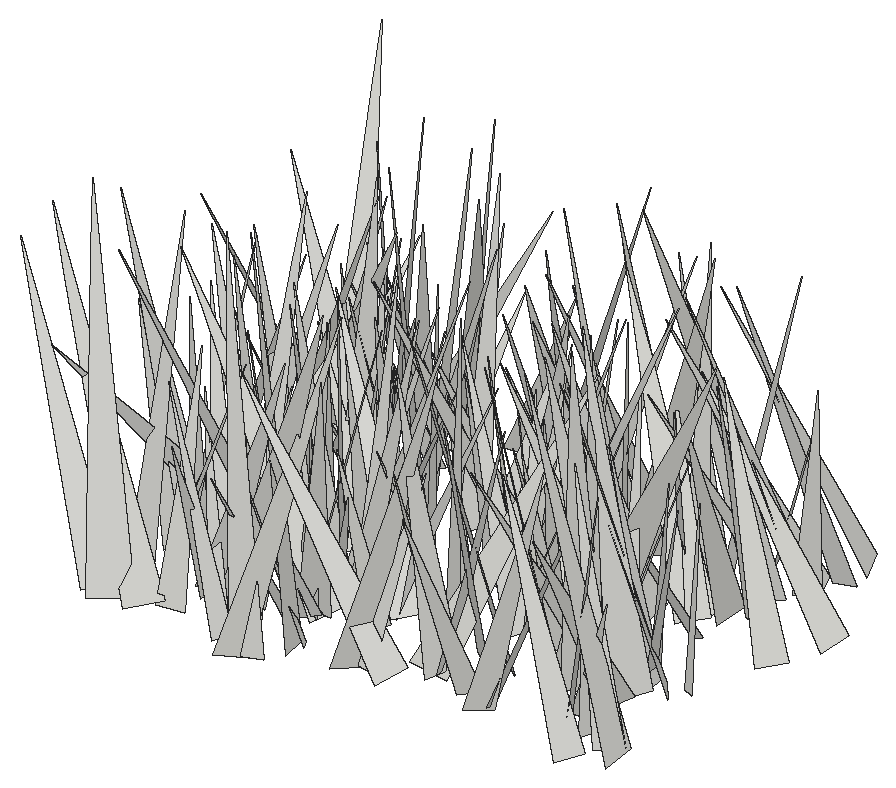
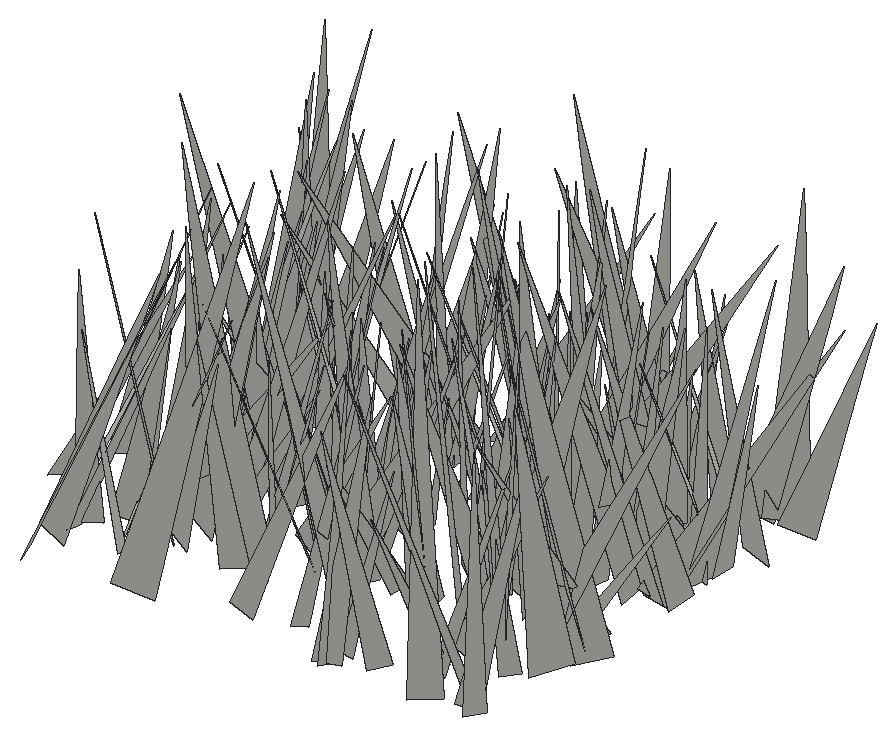
# SketchUp Ruby script. Lengths in inches.
U = 1.inch
M = Sketchup.active_model
def pt(a) = Geom::Point3d.new(a.map { |v| v * U })
def face(e, loops, mat)
  f = e.add_face(loops[0].map { |a| pt(a) })
  loops[1..].each { |l| e.add_face(l.map { |a| pt(a) }).erase! }
  f.material = f.back_material = mat if mat
  f
end
# faces: each face lists its corners as indices into pts; further lists are holes
def faces(e, pts, list, mat = nil) = list.each { |f| face(e, (f[0].is_a?(Array) ? f : [f]).map { |l| l.map { |i| pts[i] } }, mat) }
# xy, xz, yz: faces in a plane at the given z, y or x. An outline is a flat list of corners, or four numbers for a rectangle; further outlines are holes
def ring(l) = l.size == 4 ? [[l[0], l[1]], [l[2], l[1]], [l[2], l[3]], [l[0], l[3]]] : l.each_slice(2).to_a
def flat(e, list, mat, &to3) = list.each { |f| face(e, (f[0].is_a?(Array) ? f : [f]).map { |l| ring(l).map { |u, v| to3.(u, v) } }, mat) }
def xy(e, z, list, mat = nil) = flat(e, list, mat) { |x, y| [x, y, z] }
def xz(e, y, list, mat = nil) = flat(e, list, mat) { |x, z| [x, y, z] }
def yz(e, x, list, mat = nil) = flat(e, list, mat) { |y, z| [x, y, z] }
def lines(e, pts, list) = list.each { |a, b| e.add_line(pt(pts[a]), pt(pts[b])) }
# prism: a flat outline (further loops are holes) pulled along v
def prism(e, loops, v, mat = nil)
  f = face(e, loops, mat); d = Geom::Vector3d.new(v.map { |x| x * U })
  f.pushpull(f.normal.samedirection?(d) ? d.length : -d.length)
end
def box(e, o, s, mat = nil) = prism(e, [[o, [o[0] + s[0], o[1], o[2]], [o[0] + s[0], o[1] + s[1], o[2]], [o[0], o[1] + s[1], o[2]]]], [0, 0, s[2]], mat)
def at(x, y, z, deg = 0) = Geom::Transformation.translation(pt([x, y, z])) * Geom::Transformation.rotation(ORIGIN, Z_AXIS, deg.degrees)
def axes(o, x, y, z) = Geom::Transformation.new([*x, 0, *y, 0, *z, 0, *pt(o).to_a, 1])
def part(name) = M.definitions.add(name)
# library, detail: a bought-in or finely detailed component or shape, given as its bounding box
def library(name, o, s) = part(name).tap { |d| box(d.entities, o, s) }
def detail(e, o, s) = box(e.add_group.entities, o, s)
def put(e, d, t, mat = nil) = e.add_instance(d, t).tap { |i| i.material = mat if mat }
def group(e, t, mat = nil) = e.add_group.tap { |g| g.transformation = t; g.material = mat if mat }.entities
root = M.entities
c1 = part("fur_instance\#9")
p = [[0.8125,0,1.79],[0.67,-0.02,1.48],[0,-0.11,0],[0,0.11,0]]
faces(c1.entities,p,[[0,1,2,3]])
put(root,c1,axes([64.84,431.83,-27.1],[-3.24359,5.98487,0.42852],[5.75195,2.96279,2.1587],[-1.708,-1.38792,6.45597]))
put(root,c1,axes([65.26,437.11,-27.1],[-7.08698,0.49693,1.41438],[0.58095,7.2106,0.37757],[1.38199,-0.48283,7.09434]))
put(root,c1,axes([66.96,431.76,-27.1],[-3.17251,7.14398,0.8627],[6.87917,2.73438,2.65436],[-2.11131,-1.82544,7.35225]))
put(root,c1,axes([65.07,435.94,-27.1],[-4.79431,0.50788,0.77321],[0.45097,4.84644,-0.38709],[0.80772,0.30866,4.80557]))
put(root,c1,axes([65.37,445.7,-27.1],[-6.50457,4.89284,0.5628],[4.72218,6.46057,-1.59001],[1.39918,0.94188,7.98255]))
put(root,c1,axes([66.375,443.02,-27.1],[-2.80536,-2.90649,0.0794],[-2.63209,2.49174,-1.78533],[-1.23535,1.29136,3.62358]))
put(root,c1,axes([65.85,439.1,-27.1],[3.04305,-5.48081,0.27728],[-4.42438,-2.6378,-3.58374],[-3.24669,-1.54241,5.14356]))
put(root,c1,axes([65.69,431.37,-27.1],[-4.19179,6.94453,1.88873],[7.18228,4.17546,0.58769],[0.45687,-1.92457,8.09026]))
put(root,c1,axes([64.86,434.22,-27.1],[1.29784,6.7007,1.25957],[6.74597,-1.44798,0.75208],[-0.98888,-1.08363,6.78367]))
put(root,c1,axes([67.03,444.22,-27.1],[-2.83632,-6.0499,0.28173],[-5.90232,2.69141,-1.62612],[-1.35766,0.93829,6.48088]))
put(root,c1,axes([65.53,436.91,-27.1],[1.09401,4.63876,2.44173],[5.21296,-1.22556,-0.00737],[-0.55243,-2.37843,4.76601]))
put(root,c1,axes([66.2,434.94,-27.1],[3.80784,5.11048,0.67094],[4.57882,-3.73693,2.47721],[-2.36675,0.99257,5.87197]))
put(root,c1,axes([67.18,438.29,-27.1],[-2.59565,5.50063,1.7013],[5.74289,2.3395,1.19781],[-0.41302,-2.03926,5.96319]))
put(root,c1,axes([66.06,449.86,-27.1],[1.11267,-4.69864,0.20362],[-4.67497,-1.12782,-0.47895],[-0.51316,0.0867,4.80478]))
put(root,c1,axes([65.54,450.09,-27.1],[4.72712,-1.54603,0.79765],[-1.39638,-4.74943,-0.93014],[-1.03759,-0.65178,4.88576]))
put(root,c1,axes([64.83,438.68,-27.1],[6.22243,-0.20354,0.93497],[-0.30289,-6.25415,0.65425],[-0.90767,0.69164,6.19128]))
put(root,c1,axes([67.47,438.27,-27.1],[4.90342,0.51596,3.18153],[0.4361,-5.84514,0.27581],[-3.19346,-0.00597,4.92277]))
put(root,c1,axes([65.35,443.85,-27.1],[3.97347,4.57155,1.31094],[4.73936,-3.94824,-0.59665],[-0.39506,-1.38509,6.02757]))
put(root,c1,axes([65.8,442.46,-27.1],[-0.63862,5.35473,0.03552],[5.1577,0.62471,-1.44573],[1.43964,0.13724,5.19527]))
put(root,c1,axes([67.35,446.26,-27.1],[-4.34525,-4.69158,2.51984],[-5.05188,4.66036,-0.03462],[1.68493,1.87398,6.3946]))
put(root,c1,axes([68.17,439.7,-27.1],[-6.22894,0.57755,1.75246],[0.68588,6.45268,0.31131],[1.71297,-0.48351,6.24791]))
put(root,c1,axes([65.77,439.19,-27.1],[2.77668,6.00015,1.42785],[6.14966,-2.57364,-1.14395],[0.47149,-1.76779,6.51177]))
put(root,c1,axes([68.98,446.6875,-27.1],[-0.44719,-4.16584,0.88919],[-4.01944,0.11666,-1.47491],[-1.41032,0.98845,3.92158]))
put(root,c1,axes([67.33,437.82,-27.1],[-1.25475,3.57203,1.31412],[3.70812,1.4592,-0.42579],[0.858,-1.08261,3.76198]))
put(root,c1,axes([66.38,446.91,-27.1],[3.1539,-2.32332,0.00557],[-2.32207,-3.15188,0.13648],[0.07647,0.11319,3.91488]))
put(root,c1,axes([68.78,434.51,-27.1],[3.00603,-4.02582,3.59921],[-4.80148,-3.87769,-0.32715],[-2.47129,2.63706,5.01362]))
put(root,c1,axes([68.6,448.36,-27.1],[-1.93771,-4.14246,0.35212],[-4.15628,1.93921,-0.05843],[0.0961,0.34375,4.57288]))
put(root,c1,axes([67.9375,432.13,-27.1],[-1.16882,5.10436,1.64073],[5.31118,1.33199,-0.3603],[0.7334,-1.51127,5.22406]))
put(root,c1,axes([69.52,432.99,-27.1],[-0.27528,4.26527,0.41219],[4.05575,0.12601,1.40472],[-1.38323,-0.47937,4.03672]))
put(root,c1,axes([67.23,438.17,-27.1],[1.7878,3.1828,1.34143],[3.44443,-1.53093,-0.95817],[0.2561,-1.62848,3.52255]))
put(root,c1,axes([72.34,434.95,-27.1],[-3.051,-7.21191,1.32168],[-6.61753,2.09219,-3.8598],[-3.15701,2.58422,6.81338]))
put(root,c1,axes([70.76,441.16,-27.1],[-6.11884,4.72961,1.11538],[4.85918,5.97068,1.339],[0.0418,-1.7422,7.61686]))
put(root,c1,axes([67.03,435.56,-27.1],[-1.28039,5.01222,0.36244],[4.5705,1.31696,-2.06622],[2.08908,0.19072,4.74262]))
put(root,c1,axes([68.92,442.6,-27.1],[-4.7564,-0.43454,1.78324],[-0.95829,4.81251,-1.3833],[1.56539,1.62573,4.5715]))
put(root,c1,axes([64.67,444.17,-27.1],[3.10816,-7.62871,0.22312],[-7.12075,-2.81203,3.04879],[2.74626,1.34273,7.65263]))
put(root,c1,axes([68.97,437.47,-27.1],[3.31439,2.62679,2.62231],[3.03004,-3.94532,0.12232],[-2.14367,-1.5153,4.22732]))
put(root,c1,axes([67.52,445.84,-27.1],[6.90611,3.10223,2.59996],[3.46907,-7.18559,-0.64093],[-2.08547,-1.6797,7.5437]))
put(root,c1,axes([66.57,433.24,-27.1],[4.70564,3.18962,0.73071],[3.27223,-4.59158,-1.02983],[-0.01227,-1.26267,5.59072]))
put(root,c1,axes([66.61,439.19,-27.1],[7.58645,0.4489,1.20084],[0.2907,-7.62155,1.01257],[-1.24861,0.95304,7.53196]))
put(root,c1,axes([68.28,434.13,-27.1],[4.10212,-1.60455,0.85508],[-1.23063,-4.00368,-1.60913],[-1.3384,-1.23658,4.10033]))
put(root,c1,axes([70.8,431.66,-27.1],[-4.9286,0.63717,0.02707],[0.62924,4.89286,-0.60144],[0.10377,0.59304,4.93308]))
put(root,c1,axes([69.94,441.93,-27.1],[0.78619,5.10987,0.99795],[4.99569,-1.02461,1.31074],[-1.46621,-0.75112,5.00108]))
put(root,c1,axes([69.4,439.2,-27.1],[-3.39336,2.50243,2.08506],[2.97495,3.60715,0.51243],[1.32637,-1.68843,4.18502]))
put(root,c1,axes([72.78,435.59,-27.1],[-6.95314,3.37085,0.59923],[3.40426,6.66259,2.02209],[-0.36434,-2.07731,7.45788]))
put(root,c1,axes([66.53,449.09,-27.1],[3.98085,5.13777,1.04709],[4.9615,-3.26572,-2.83883],[1.69606,-2.50573,5.84679]))
put(root,c1,axes([68.85,447.96,-27.1],[-0.53064,3.51066,0.60828],[3.36851,0.69471,-1.0709],[1.16098,-0.41106,3.38519]))
put(root,c1,axes([71.38,439.95,-27.1],[-4.19942,1.95994,0.17006],[1.96728,4.18576,0.33862],[0.01038,-0.37878,4.62189]))
put(root,c1,axes([69.54,447.65,-27.1],[4.78863,4.89843,2.46119],[5.13986,-5.14824,0.24599],[-1.90629,-1.57608,6.84581]))
put(root,c1,axes([70.67,439.91,-27.1],[-2.92778,3.00983,0.00711],[2.98882,2.90849,-0.48849],[0.35507,0.33555,4.17041]))
put(root,c1,axes([69.49,441.11,-27.1],[6.01123,-4.10409,2.83515],[-4.50522,-6.3728,0.32708],[-2.14119,1.8869,7.27128]))
put(root,c1,axes([70.33,442.76,-27.1],[-1.26664,-5.03308,1.07763],[-5.14261,1.28411,-0.04714],[0.2163,1.05675,5.1898]))
put(root,c1,axes([70.47,433.3,-27.1],[0.64716,8.27924,1.09317],[8.31403,-0.74193,0.69715],[-0.78591,-1.0312,8.27518]))
put(root,c1,axes([70.23,441.09,-27.1],[-1.89592,-3.45095,1.30694],[-3.60556,2.04518,0.16982],[0.78554,1.05823,3.9338]))
put(root,c1,axes([67.71,450.3,-27.1],[7.63705,-2.12328,0.08153],[-2.0044,-7.29978,-2.35267],[-0.70524,-2.24596,7.56953]))
put(root,c1,axes([70.04,439.05,-27.1],[-2.18081,-4.36379,1.96245],[-4.63729,2.45895,0.31456],[1.17875,1.60022,4.86823]))
put(root,c1,axes([68.3,434.26,-27.1],[3.9818,-4.86666,0.84742],[-4.90357,-3.76221,1.43455],[0.59785,1.55519,6.12218]))
put(root,c1,axes([69.31,446.01,-27.1],[-4.14785,-5.45032,3.6874],[-5.74845,5.12259,1.10541],[3.20285,2.13555,6.75935]))
put(root,c1,axes([71.05,437.95,-27.1],[1.22573,-5.85041,2.29876],[-6.17569,-1.55733,-0.67049],[-1.1715,2.08841,5.93971]))
put(root,c1,axes([72.45,431.02,-27.1],[0.0482,8.00911,1.76337],[7.92916,-0.49572,2.03478],[-2.09374,-1.69294,7.74648]))
put(root,c1,axes([72.39,438.34,-27.1],[-5.98582,-0.44068,0.88109],[-0.67667,5.78235,-1.70504],[0.71598,1.78068,5.75475]))
put(root,c1,axes([70.06,440.17,-27.1],[-4.21577,-3.58718,3.5566],[-4.31781,4.96325,-0.11214],[2.62178,2.40587,5.53425]))
put(root,c1,axes([70.68,437.94,-27.1],[-2.8459,-6.01928,1.64103],[-5.98512,3.14324,1.14988],[1.76154,0.95508,6.5581]))
put(root,c1,axes([70.69,442.29,-27.1],[1.15457,-5.41906,0.82486],[-5.48032,-1.12384,0.28761],[0.11275,0.86626,5.53322]))
put(root,c1,axes([72.46,433.89,-27.1],[-0.70477,-3.63934,0.22038],[-3.52996,0.62491,-0.96896],[-0.91253,0.39339,3.57807]))
put(root,c1,axes([71.88,444.66,-27.1],[4.93577,0.48548,2.66433],[-0.37318,-5.36398,1.66873],[-2.68236,1.63958,4.67042]))
put(root,c1,axes([70.28,437.95,-27.1],[5.04239,2.3615,1.06864],[2.46365,-5.09289,-0.37039],[-0.80566,-0.79378,5.55564]))
put(root,c1,axes([73.37,432.68,-27.1],[-7.60319,-2.30719,2.08818],[-2.71089,7.61771,-1.45385],[1.52798,2.03457,7.8114]))
put(root,c1,axes([72,442.17,-27.1],[-6.4664,-4.252,2.80304],[-4.40658,6.94256,0.3657],[2.55316,1.21333,7.73047]))
put(root,c1,axes([69.96,443.15,-27.1],[5.00049,1.26706,0.71261],[1.41038,-4.84715,-1.27832],[-0.35226,-1.4205,4.99762]))
put(root,c1,axes([71,438.52,-27.1],[5.57047,2.74276,2.66238],[3.42235,-5.67452,-1.31471],[-1.7025,-2.43273,6.06831]))
put(root,c1,axes([71.38,436.54,-27.1],[2.3019,2.88607,2.09295],[3.52279,-2.224,-0.8077],[-0.54756,-2.17555,3.60219]))
put(root,c1,axes([72.13,449.54,-27.1],[-0.71572,-3.67555,0.46048],[-3.70429,0.70984,-0.09154],[-0.00255,0.46948,3.74347]))
put(root,c1,axes([72.99,443.83,-27.1],[-6.34351,2.24327,1.15963],[1.89857,6.30395,-1.80908],[1.66506,1.35834,6.48071]))
put(root,c1,axes([71.18,442.35,-27.1],[5.70541,0.17051,1.69377],[-0.31532,-5.71566,1.63753],[-1.67287,1.65887,5.46803]))
put(root,c1,axes([73.53,433.14,-27.1],[-3.08913,-1.9262,0.20442],[-1.91689,2.98464,-0.84391],[-0.27849,0.82245,3.5413]))
put(root,c1,axes([70.51,449.5,-27.1],[2.89103,-3.61881,0.35286],[-3.55779,-2.72252,1.22815],[0.74997,1.03461,4.46604]))
put(root,c1,axes([71.47,438.4375,-27.1],[3.13584,4.70476,0.63652],[4.72939,-3.16238,0.0748],[-0.41563,-0.48786,5.65355]))
put(root,c1,axes([69.64,434.24,-27.1],[3.88235,-7.18309,1.19208],[-7.15051,-3.50623,2.16032],[1.37403,2.04942,7.87416]))
put(root,c1,axes([71.15,441.0625,-27.1],[4.07736,0.20577,0.16386],[0.20057,-4.0788,0.13116],[-0.17019,0.12285,4.08044]))
put(root,c1,axes([71.92,435.21,-27.1],[2.13967,5.72529,2.72362],[6.33838,-1.99885,-0.77766],[-0.14822,-2.82858,6.06237]))
put(root,c1,axes([75.21,437.24,-27.1],[-4.13597,4.87198,0.25098],[4.78591,3.98836,1.44689],[-0.94567,-1.12348,6.22487]))
put(root,c1,axes([72.26,450.47,-27.1],[3.35364,-3.87615,0.32814],[-3.76663,-3.34394,-1.00479],[-0.97195,-0.41544,5.02611]))
put(root,c1,axes([72.58,441.81,-27.1],[-3.23296,-4.09809,2.47034],[-4.47809,3.64184,0.18098],[1.68632,1.81429,5.21667]))
put(root,c1,axes([71.93,430.74,-27.1],[6.32729,-2.1008,2.73388],[-3.01636,-6.1404,2.26257],[-1.67006,3.13117,6.27127]))
put(root,c1,axes([73.9,436.03,-27.1],[1.51119,6.34193,0.92742],[6.21067,-1.68435,1.39797],[-1.58356,-0.55387,6.36784]))
put(root,c1,axes([71.85,438.29,-27.1],[4.96936,4.425,0.65774],[4.44372,-4.99597,0.03757],[-0.51632,-0.4092,6.65385]))
put(root,c1,axes([72.25,450.61,-27.1],[5.97611,0.87511,2.00016],[1.66713,-5.59279,-2.53411],[-1.40966,-2.90435,5.48252]))
put(root,c1,axes([72.27,435.28,-27.1],[1.6892,-5.96403,1.00433],[-6.01842,-1.55459,0.89085],[0.59746,1.20222,6.13428]))
put(root,c1,axes([72.22,436.71,-27.1],[-0.71595,-3.844,0.50308],[-3.36107,0.87042,1.86752],[1.93201,0.08975,3.4353]))
put(root,c1,axes([73.64,444.34,-27.1],[-2.96386,2.60362,0.59977],[2.15648,2.85999,-1.75873],[1.5774,0.98217,3.53132]))
put(root,c1,axes([74.78,444.54,-27.1],[-4.80536,-1.45342,1.08645],[-0.98448,4.67157,1.89512],[1.52434,-1.5647,4.64891]))
put(root,c1,axes([77.17,442.39,-27.1],[-0.65869,-6.64833,1.3688],[-6.16249,0.00919,-2.92087],[-2.84565,1.51902,6.00855]))
put(root,c1,axes([77.55,433.24,-27.1],[-6.03456,2.61232,0.13904],[2.52964,5.73798,1.98392],[-0.66667,-1.87372,6.2693]))
put(root,c1,axes([75.55,440.27,-27.1],[-3.65849,-0.26653,0.63033],[-0.40108,3.61269,-0.80033],[0.55452,0.85461,3.57982]))
put(root,c1,axes([74.94,435.78,-27.1],[3.15907,-2.58161,1.45094],[-2.40771,-3.47422,-0.93937],[-1.72421,0.12146,3.97014]))
put(root,c1,axes([73.4,436.375,-27.1],[2.35807,6.09522,2.44102],[6.53945,-1.94795,-1.45322],[0.58808,-2.77931,6.37184]))
put(root,c1,axes([74.79,448.91,-27.1],[4.72297,-1.05883,1.70864],[-0.28791,-4.67444,-2.10088],[-1.98939,-1.83725,4.36049]))
put(root,c1,axes([75.84,438.59,-27.1],[-3.61169,-1.5954,0.61372],[-1.41522,3.59542,1.01805],[0.9587,-0.70282,3.81487]))
put(root,c1,axes([76.19,441.05,-27.1],[-1.43157,-3.77915,1.63266],[-4.11341,1.2436,-0.72817],[-0.16553,1.78,3.97506]))
put(root,c1,axes([77.23,449.33,-27.1],[-0.62326,-5.57048,0.69706],[-5.46922,0.44429,-1.33972],[-1.26641,0.82277,5.44278]))
put(root,c1,axes([73.93,447.18,-27.1],[7.81228,1.65656,1.00866],[1.73052,-7.84393,-0.52089],[-0.87571,-0.72239,7.96898]))
put(root,c1,axes([77.86,435.82,-27.1],[-5.58164,-0.15602,0.84627],[-0.25003,5.60842,-0.61509],[0.82341,0.64537,5.54984]))
put(root,c1,axes([77.59,447.72,-27.1],[-4.87581,-1.54153,0.97742],[-1.54685,4.96967,0.12147],[0.96896,0.17664,5.11224]))
put(root,c1,axes([77.79,440.65,-27.1],[1.94279,3.86541,2.10519],[3.74501,-2.66073,1.42935],[-2.3126,-1.06149,4.08323]))
put(root,c1,axes([78.6,443.92,-27.1],[-1.09532,-3.977,1.33167],[-3.82769,0.38536,-1.99748],[-1.71426,1.68065,3.6092]))
put(root,c1,axes([74.32,437.46,-27.1],[4.41432,4.17138,0.78555],[4.1779,-4.06951,-1.86761],[0.75011,-1.88212,5.77916]))
put(root,c1,axes([77.64,441,-27.1],[-3.40834,-0.81843,0.94444],[-0.85751,3.5273,-0.03792],[0.90911,0.25869,3.50503]))
put(root,c1,axes([79.24,438.75,-27.1],[-5.48361,2.04542,0.49712],[2.0602,5.49974,0.09665],[0.43181,-0.2646,5.85187]))
put(root,c1,axes([76.24,433.11,-27.1],[-0.49271,4.25835,1.65602],[4.30491,0.99075,-1.26683],[1.53091,-1.41548,4.0953]))
put(root,c1,axes([75.44,444.21,-27.1],[0.87943,-6.58228,1.27772],[-6.45662,-0.48373,1.95201],[1.80858,1.47376,6.34739]))
put(root,c1,axes([80.11,444.08,-27.1],[-7.13799,-1.18277,0.6594],[-1.323,6.84565,-2.04241],[0.28881,2.12669,6.94107]))
put(root,c1,axes([77.62,444.34,-27.1],[2.96652,3.66752,1.13191],[3.55325,-3.16507,0.94281],[-1.45132,-0.25254,4.62191]))
put(root,c1,axes([77.86,441.44,-27.1],[-3.21218,-2.63282,1.4726],[-2.81239,3.39173,-0.07071],[1.09119,0.99138,4.15269]))
put(root,c1,axes([75.89,432.79,-27.1],[6.31096,-2.97385,1.65761],[-3.28181,-6.24286,1.29466],[-0.9062,1.89806,6.85536]))
put(root,c1,axes([78.66,441.64,-27.1],[-2.98771,2.56269,0.00271],[2.54357,2.96592,-0.47684],[0.31249,0.36018,3.90722]))
put(root,c1,axes([77.93,435.79,-27.1],[-3.99319,-2.60087,1.40659],[-2.16034,4.18012,1.59628],[2.0189,-0.6713,4.49021]))
put(root,c1,axes([78.68,440.01,-27.1],[-1.71851,4.03919,1.0736],[4.16688,1.74577,0.10182],[0.32374,-1.02868,4.3884]))
put(root,c1,axes([78.78,435.31,-27.1],[2.86323,5.98862,2.41998],[6.20716,-3.28322,0.78076],[-1.78634,-1.80966,6.59182]))
put(root,c1,axes([78.86,434.67,-27.1],[-5.74569,2.33772,2.68731],[2.89131,6.03979,0.92776],[2.08013,-1.9379,6.13328]))
put(root,c1,axes([78.98,445.25,-27.1],[3.80015,2.05854,2.10545],[1.83657,-4.34391,0.93228],[-2.30164,-0.0674,4.22014]))
put(root,c1,axes([77.28,445.0625,-27.1],[4.12664,4.96749,0.53315],[4.97839,-4.14664,0.10195],[-0.41933,-0.34468,6.45715]))
put(root,c1,axes([78.79,439.1,-27.1],[1.97963,5.14738,0.61551],[5.06452,-2.06097,0.94673],[-1.10678,-0.22402,5.43306]))
put(root,c1,axes([80.59,436.52,-27.1],[-4.6315,-5.30606,1.24554],[-5.44783,4.55599,-0.84886],[0.16366,1.49838,6.99175]))
put(root,c1,axes([78.07,443.45,-27.1],[4.2644,-2.86076,0.08373],[-2.8192,-4.22473,-0.76148],[-0.49304,-0.58632,5.07831]))
put(root,c1,axes([77.3,441.98,-27.1],[4.68379,1.41709,0.13919],[1.37897,-4.39495,-1.65779],[0.35492,-1.62533,4.60411]))
put(root,c1,axes([78.77,434.95,-27.1],[5.20805,0.62891,1.21236],[0.54515,-5.33937,0.42794],[-1.25226,0.29119,5.2284]))
put(root,c1,axes([77.29,441.31,-27.1],[6.01088,3.96881,0.98389],[4.08835,-5.80352,-1.56674],[0.06989,-1.84874,7.03046]))
put(root,c1,axes([79.42,446.98,-27.1],[-2.32023,4.26891,1.78267],[4.38145,2.66784,-0.68595],[1.48474,-1.20167,4.81004]))
put(root,c1,axes([79.625,436.14,-27.1],[-2.94569,-5.43055,1.36405],[-5.282,3.20651,1.35919],[1.85796,0.50597,6.02666]))
put(root,c1,axes([81.87,443.4,-27.1],[-2.56697,2.61634,0.35758],[2.51502,2.27032,1.44317],[-0.80484,-1.25014,3.36925]))
put(root,c1,axes([82.54,446.58,-27.1],[0.67019,6.07953,1.22269],[5.42193,-1.17133,2.85227],[-3.0097,-0.75637,5.41058]))
put(root,c1,axes([79.81,440.3,-27.1],[-0.67343,-4.75938,1.30258],[-4.88536,0.82798,0.49956],[0.69398,1.21023,4.78075]))
put(root,c1,axes([80.6,434.1,-27.1],[1.77342,-4.13167,0.71101],[-4.001,-1.89854,-1.053],[-1.2523,0.21471,4.37115]))
put(root,c1,axes([80.79,439.76,-27.1],[-3.85431,-2.63258,1.04926],[-2.43046,3.98156,1.06172],[1.4575,-0.32233,4.54521]))
put(root,c1,axes([81.27,450.75,-27.1],[1.71301,-8.16044,0.92704],[-8.06805,-1.84913,-1.36891],[-1.53583,0.61199,8.22516]))
put(root,c1,axes([78.37,434.41,-27.1],[-2.47927,6.31853,1.78834],[5.49074,3.04318,-3.14001],[3.60191,-0.28983,6.01756]))
put(root,c1,axes([82.39,445.32,-27.1],[1.71463,6.79892,3.94816],[7.36353,-2.80488,1.63226],[-2.7553,-3.26505,6.81916]))
put(root,c1,axes([77.51,442.77,-27.1],[5.84897,4.9177,0.90335],[4.92852,-5.43629,-2.31659],[0.84231,-2.33947,7.282]))
put(root,c1,axes([82.76,440.5,-27.1],[-6.27523,-0.24227,0.55286],[-0.1392,6.19931,1.13667],[0.58735,-1.11924,6.17618]))
put(root,c1,axes([81.25,438.75,-27.1],[0.8668,-4.44855,1.11397],[-4.54098,-0.99091,-0.42373],[-0.6404,1.00517,4.51236]))
put(root,c1,axes([82.95,436.62,-27.1],[-4.95008,-4.07189,1.35786],[-4.2827,4.82407,-1.14641],[0.2873,1.75371,6.30629]))
put(root,c1,axes([84.01,446.89,-27.1],[-6.46685,-0.99912,0.02995],[-0.985,6.33639,-1.3035],[-0.17003,1.29271,6.41243]))
put(root,c1,axes([82.32,442.85,-27.1],[-6.75805,0.02177,1.99006],[0.56326,6.77748,1.83863],[1.90881,-1.92284,6.50317]))
put(root,c1,axes([83.66,443.71,-27.1],[-6.02819,4.2729,0.70004],[4.32885,5.97346,0.81585],[0.09372,-1.07093,7.34378]))
put(root,c1,axes([79.28,446.29,-27.1],[6.86151,-4.43995,0.81428],[-4.49635,-6.85344,0.51929],[-0.39875,0.87961,8.15621]))
put(root,c1,axes([81.89,439.34,-27.1],[-4.9139,-3.74374,0.55427],[-3.15126,4.55055,2.79845],[2.0958,-1.9355,5.50733]))
put(root,c1,axes([84.58,442.65,-27.1],[-2.08934,-4.39389,0.06996],[-3.98317,1.86084,-2.08523],[-1.85622,0.95264,4.39584]))
put(root,c1,axes([82.84,444.71,-27.1],[0.75585,6.87514,1.87347],[7.05211,-0.99202,0.79528],[-1.02238,-1.75986,6.87069]))
put(root,c1,axes([83.77,443.71,-27.1],[-3.58743,2.64736,0.43412],[2.66538,3.59954,0.07504],[0.30449,-0.3184,4.45786]))
put(root,c1,axes([81.83,433.81,-27.1],[5.28462,2.45266,0.54887],[2.09175,-5.00051,2.20534],[-1.39334,1.79538,5.39252]))
put(root,c1,axes([84.27,438.82,-27.1],[0.39127,5.5531,0.09038],[5.24022,-0.39914,1.8382],[-1.83989,0.04412,5.25462]))
put(root,c1,axes([83.51,438.73,-27.1],[3.66547,-5.8791,2.24711],[-5.89364,-4.11869,-1.16204],[-2.20868,1.23351,6.83002]))
put(root,c1,axes([82.16,444.88,-27.1],[-2.28168,-4.43341,1.38047],[-4.1851,2.6298,1.52839],[2.0114,0.44265,4.74608]))
put(root,c1,axes([81.66,433.32,-27.1],[4.65487,-3.05281,1.35089],[-3.29302,-4.57961,0.99778],[-0.54826,1.58741,5.47649]))
put(root,c1,axes([84.18,447.56,-27.1],[-4.88167,-3.98465,0.29136],[-3.56929,4.55624,2.50876],[1.79514,-1.77658,5.7805]))
put(root,c1,axes([82.6,437.08,-27.1],[0.98375,-3.96673,0.69714],[-3.91068,-0.76919,1.14174],[0.96305,0.9285,3.92417]))
put(root,c1,axes([82.75,446.63,-27.1],[4.81614,4.80746,1.57054],[5.00941,-4.83285,-0.56818],[-0.69571,-1.51836,6.78115]))
put(root,c1,axes([86.23,450.9375,-27.1],[-6.15592,-2.89241,0.11132],[-2.84807,6.09927,0.98037],[0.51666,-0.84058,6.73054]))
put(root,c1,axes([83.8125,437.93,-27.1],[3.6245,2.89722,0.22495],[2.66528,-3.45765,1.58821],[-1.15791,1.11007,4.35987]))
put(root,c1,axes([80.59,441.95,-27.1],[3.82613,-7.13137,0.63835],[-6.75778,-3.35774,2.99351],[2.36564,1.94225,7.51895]))
put(root,c1,axes([84.66,437.6,-27.1],[-2.85824,2.70123,1.97363],[3.21945,2.92659,0.65696],[0.90938,-1.87078,3.87745]))
put(root,c1,axes([85.58,438.92,-27.1],[-4.70558,-0.80345,0.83315],[-0.88013,4.74917,-0.39105],[0.7517,0.53106,4.75763]))
put(root,c1,axes([86.35,449.2,-27.1],[-1.63613,-6.00923,1.56488],[-6.02721,1.14742,-1.89548],[-1.49415,1.95172,5.93253]))
put(root,c1,axes([86.01,448.29,-27.1],[-6.75502,-2.37628,0.59319],[-2.11002,6.52988,2.13012],[1.24354,-1.82836,6.83664]))
put(root,c1,axes([84.92,446.59,-27.1],[1.57492,-4.967,1.49516],[-5.0252,-1.8484,-0.84719],[-1.28605,1.13987,5.14138]))
put(root,c1,axes([84.68,440.13,-27.1],[-3.9391,-6.11846,0.96009],[-6.01065,4.05101,1.1555],[1.49311,0.1661,7.18449]))
put(root,c1,axes([86.24,438.79,-27.1],[-5.08924,-4.37631,0.84531],[-4.44671,5.07308,-0.50754],[0.30556,0.93743,6.69289]))
put(root,c1,axes([83.85,436.85,-27.1],[3.80262,-6.94068,2.14426],[-7.19034,-3.9408,-0.00453],[-1.0344,1.87826,7.9141]))
put(root,c1,axes([85.44,437.625,-27.1],[-6.5147,3.53544,2.59254],[3.94464,6.75335,0.70282],[1.91322,-1.88542,7.3788]))
put(root,c1,axes([86.06,434.5625,-27.1],[-7.47088,0.3057,1.86762],[-0.12287,7.51123,-1.721],[1.88848,1.69808,7.27638]))
put(root,c1,axes([86.57,432.55,-27.1],[-4.85696,2.92878,0.85344],[3.03677,4.79447,0.82904],[0.29007,-1.15391,5.61075]))
put(root,c1,axes([87.12,446.99,-27.1],[-4.6266,-2.97065,0.07987],[-2.96143,4.59663,-0.58091],[-0.24706,0.53178,5.46742]))
put(root,c1,axes([85.47,444.83,-27.1],[-2.10468,-4.52268,1.53831],[-4.75533,2.14388,-0.20306],[0.45584,1.48319,4.98428]))
put(root,c1,axes([83.5,448.6,-27.1],[4.06757,1.21437,0.51699],[1.31683,-3.847,-1.32426],[-0.08902,-1.4188,4.03313]))
put(root,c1,axes([84.55,444.67,-27.1],[5.34642,-2.10558,1.0321],[-1.67954,-5.23165,-1.97278],[-1.63641,-1.50973,5.39684]))
put(root,c1,axes([84.96,439.65,-27.1],[4.07501,0.67414,1.38281],[0.80205,-4.27202,-0.28088],[-1.31276,-0.5174,4.12083]))
put(root,c1,axes([85.42,436.97,-27.1],[4.02503,-3.95124,0.17731],[-3.62061,-3.78264,-2.10414],[-1.59215,-1.38705,5.23314]))
put(root,c1,axes([88.13,445.88,-27.1],[-6.75441,-2.93713,0.31923],[-2.94167,6.75982,-0.04619],[0.27431,0.1697,7.36523]))
put(root,c1,axes([87.99,433.68,-27.1],[-7.83982,-0.95667,1.33619],[-0.96404,7.9519,0.03699],[1.33088,0.12461,7.89789]))
put(root,c1,axes([85.69,433.46,-27.1],[4.582,2.26461,1.64468],[2.3704,-4.81752,0.02956],[-1.48816,-0.70087,5.111]))
put(root,c1,axes([84.92,435.28,-27.1],[1.46313,-3.34357,0.17988],[-3.25058,-1.37123,0.95187],[0.80348,0.54115,3.52337]))
put(root,c1,axes([85.29,438.92,-27.1],[4.21688,0.53755,0.91963],[0.65776,-4.26755,-0.52159],[-0.83787,-0.64478,4.21888]))
put(root,c1,axes([87.31,434,-27.1],[1.60632,-4.77246,2.92285],[-5.28453,-2.29441,-0.84211],[-1.84207,2.42054,4.96463]))
put(root,c1,axes([88.9,445.43,-27.1],[-5.72955,1.74546,0.28048],[1.75274,5.48455,1.67353],[-0.23061,-1.68113,5.75097]))
put(root,c1,axes([85.82,447.64,-27.1],[2.40691,-4.24835,1.2679],[-4.42272,-2.4014,0.34948],[-0.30924,1.27831,4.87028]))
put(root,c1,axes([86.93,439.16,-27.1],[1.67627,3.15128,1.04901],[3.10636,-1.90337,0.75402],[-1.17538,-0.53615,3.48882]))
put(root,c1,axes([88.05,442.73,-27.1],[-4.17135,3.80631,1.04328],[3.93898,4.10999,0.75433],[0.24669,-1.26356,5.59635]))
